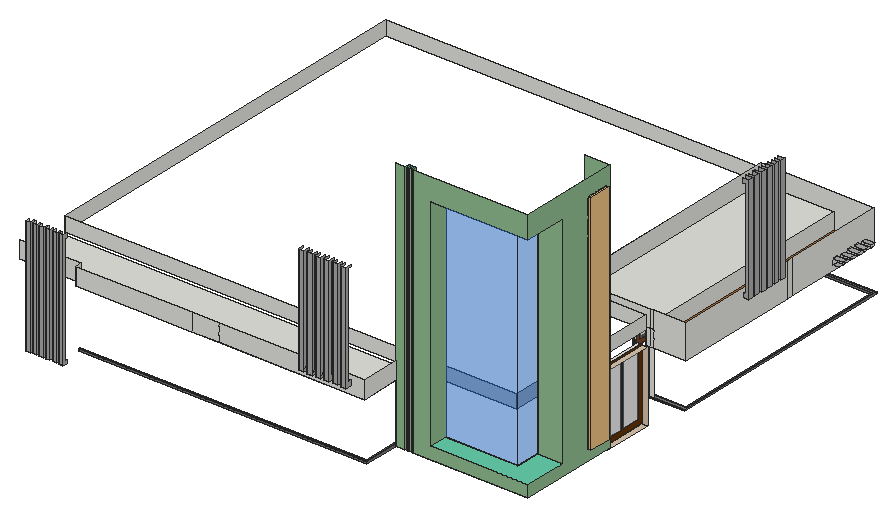
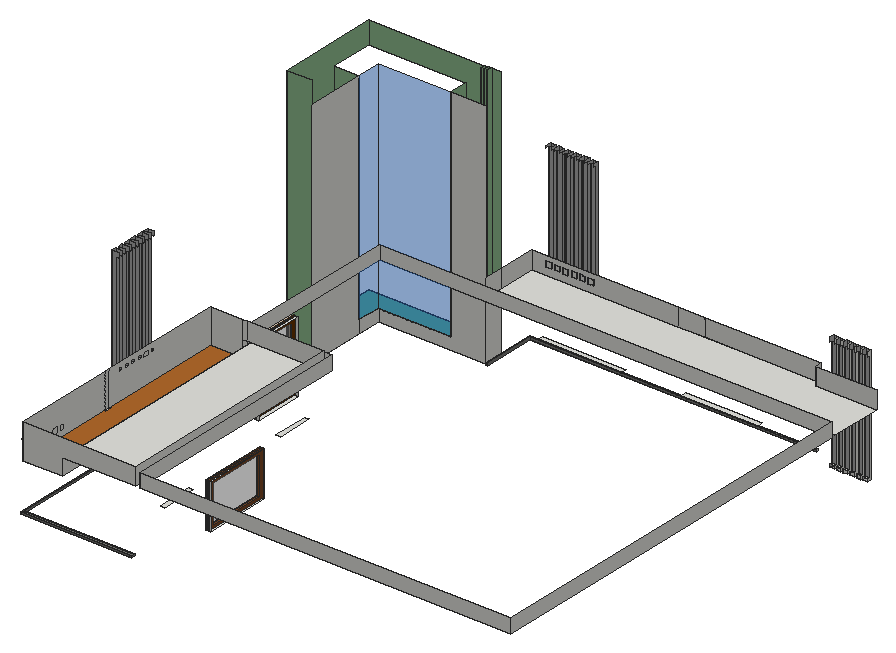
# SketchUp Ruby script. Lengths in inches.
U = 1.inch
M = Sketchup.active_model
def pt(a) = Geom::Point3d.new(a.map { |v| v * U })
def face(e, loops, mat)
  f = e.add_face(loops[0].map { |a| pt(a) })
  loops[1..].each { |l| e.add_face(l.map { |a| pt(a) }).erase! }
  f.material = f.back_material = mat if mat
  f
end
# faces: each face lists its corners as indices into pts; further lists are holes
def faces(e, pts, list, mat = nil) = list.each { |f| face(e, (f[0].is_a?(Array) ? f : [f]).map { |l| l.map { |i| pts[i] } }, mat) }
# xy, xz, yz: faces in a plane at the given z, y or x. An outline is a flat list of corners, or four numbers for a rectangle; further outlines are holes
def ring(l) = l.size == 4 ? [[l[0], l[1]], [l[2], l[1]], [l[2], l[3]], [l[0], l[3]]] : l.each_slice(2).to_a
def flat(e, list, mat, &to3) = list.each { |f| face(e, (f[0].is_a?(Array) ? f : [f]).map { |l| ring(l).map { |u, v| to3.(u, v) } }, mat) }
def xy(e, z, list, mat = nil) = flat(e, list, mat) { |x, y| [x, y, z] }
def xz(e, y, list, mat = nil) = flat(e, list, mat) { |x, z| [x, y, z] }
def yz(e, x, list, mat = nil) = flat(e, list, mat) { |y, z| [x, y, z] }
def lines(e, pts, list) = list.each { |a, b| e.add_line(pt(pts[a]), pt(pts[b])) }
# prism: a flat outline (further loops are holes) pulled along v
def prism(e, loops, v, mat = nil)
  f = face(e, loops, mat); d = Geom::Vector3d.new(v.map { |x| x * U })
  f.pushpull(f.normal.samedirection?(d) ? d.length : -d.length)
end
def box(e, o, s, mat = nil) = prism(e, [[o, [o[0] + s[0], o[1], o[2]], [o[0] + s[0], o[1] + s[1], o[2]], [o[0], o[1] + s[1], o[2]]]], [0, 0, s[2]], mat)
def at(x, y, z, deg = 0) = Geom::Transformation.translation(pt([x, y, z])) * Geom::Transformation.rotation(ORIGIN, Z_AXIS, deg.degrees)
def axes(o, x, y, z) = Geom::Transformation.new([*x, 0, *y, 0, *z, 0, *pt(o).to_a, 1])
def part(name) = M.definitions.add(name)
# library, detail: a bought-in or finely detailed component or shape, given as its bounding box
def library(name, o, s) = part(name).tap { |d| box(d.entities, o, s) }
def detail(e, o, s) = box(e.add_group.entities, o, s)
def put(e, d, t, mat = nil) = e.add_instance(d, t).tap { |i| i.material = mat if mat }
def group(e, t, mat = nil) = e.add_group.tap { |g| g.transformation = t; g.material = mat if mat }.entities
root = M.entities
M.materials.add("[0072_DarkSeaGreen]").color = [143, 188, 143]
M.materials.add("[0086_MediumAquamarine]").color = [102, 205, 170]
M.materials.add("[Blinds Cellular White]").color = [216, 195, 171]
M.materials.add("[Color C08]").color = [102, 51, 0]
M.materials.add("[Color E02]").color = [255, 255, 153]
M.materials.add("[Color M03]").color = [170, 170, 170]
M.materials.add("[Metal Seamed]").color = [118, 119, 115]
M.materials.add("[Translucent Glass Gray]").color = [128, 128, 128]
M.materials["[Translucent Glass Gray]"].alpha = 0.5
M.materials.add("[Translucent Glass Sky Reflection]").color = [37, 119, 229]
M.materials["[Translucent Glass Sky Reflection]"].alpha = 0.52
M.materials.add("[Wood Bamboo]").color = [177, 105, 43]
M.materials.add("[Wood Veneer 01]").color = [120, 70, 37]
c1 = part("Group\#4")
xy(c1.entities,0,[[0,0,92.3125,1154.125]],"[Wood Veneer 01]")
xy(c1.entities,74.3,[[0,74.3,92.3125,1079.83]],"[Wood Veneer 01]")
xy(c1.entities,936.58,[[0,74.3,92.3125,1079.83]],"[Wood Veneer 01]")
xy(c1.entities,1010.875,[[0,0,92.3125,1154.125]],"[Wood Veneer 01]")
xz(c1.entities,0,[[0,0,92.3125,1010.875]],"[Wood Veneer 01]")
xz(c1.entities,74.3,[[0,74.3,92.3125,936.58]],"[Wood Veneer 01]")
xz(c1.entities,1079.83,[[0,74.3,92.3125,936.58]],"[Wood Veneer 01]")
xz(c1.entities,1154.125,[[0,0,92.3125,1010.875]],"[Wood Veneer 01]")
yz(c1.entities,0,[[[0,0,1154.125,1010.875],[74.3,74.3,1079.83,936.58]]],"[Wood Veneer 01]")
yz(c1.entities,92.3125,[[74.3,74.3,1079.83,936.58]],"[Translucent Glass Gray]")
yz(c1.entities,92.3125,[[[0,0,1154.125,1010.875],[74.3,74.3,1079.83,936.58]]],"[Wood Veneer 01]")
c2 = part("Group\#1")
xy(c2.entities,0,[[0,0,56.25,1.4375]],"[Color C08]")
xy(c2.entities,4.61,[[4.61,0,27.19,1.4375],[28.74,0,51.64,1.4375]],"[Color C08]")
xy(c2.entities,68.58,[[4.61,0,27.19,1.4375],[28.74,0,51.64,1.4375]],"[Color C08]")
xy(c2.entities,73.1875,[[0,0,56.25,1.4375]],"[Color C08]")
xz(c2.entities,0,[[[0,0,56.25,73.1875],[28.74,4.61,51.64,68.58],[4.61,4.61,27.19,68.58]]],"[Color C08]")
xz(c2.entities,0,[[4.61,4.61,27.19,68.58],[28.74,4.61,51.64,68.58]],"[Translucent Glass Gray]")
xz(c2.entities,1.4375,[[[0,0,56.25,73.1875],[28.74,4.61,51.64,68.58],[4.61,4.61,27.19,68.58]]],"[Color C08]")
yz(c2.entities,0,[[0,0,1.4375,73.1875]],"[Color C08]")
yz(c2.entities,4.61,[[0,4.61,1.4375,68.58]],"[Color C08]")
yz(c2.entities,27.19,[[0,4.61,1.4375,68.58]],"[Color C08]")
yz(c2.entities,28.74,[[0,4.61,1.4375,68.58]],"[Color C08]")
yz(c2.entities,51.64,[[0,4.61,1.4375,68.58]],"[Color C08]")
yz(c2.entities,56.25,[[0,0,1.4375,73.1875]],"[Color C08]")
c3 = library("D E S H M U K H",[0.1875,0,0],[29.86,305.5625,4])
xy(root,172.67,[[554.1875,452.44,560.1875,543.38]])
xy(root,173.05,[[663.6875,257.99,669.6875,324.49]])
xy(root,173.05,[[669.6875,257.99,676.75,324.49]],"[Blinds Cellular White]")
xy(root,180.1,[[70.8125,30.88,76.8125,36.13],[79.75,30.88,85.75,36.07],[88.6875,30.88,94.6875,35.88],[97.625,30.88,103.625,36.25],[106.5625,30.88,112.5625,36.13],
  [115.375,30.88,121.375,36.13]],"[Color M03]")
xy(root,184.32,[[70.8125,33.13,76.8125,36.13],[79.75,33.13,85.75,36.07],[88.6875,33.13,94.6875,35.88],[97.625,33.13,103.625,36.25],[106.5625,33.13,112.5625,36.13],
  [115.375,33.13,121.375,36.13]])
xy(root,194,[[663.6875,344.5,663.6875,349.5,708.8125,349.5,708.8125,663.625,560.1875,663.625,560.1875,668.5625,711.3125,668.5625,711.3125,344.5]],"[Metal Seamed]")
xy(root,196,[[663.6875,344.5,711.3125,344.5,711.3125,668.5625,560.1875,668.5625,560.1875,663.625,708.8125,663.625,708.8125,349.5,663.6875,349.5]],"[Metal Seamed]")
xy(root,197.41,[[133.9375,41,133.9375,43,521.9375,43,521.9375,114.75,523.9375,114.75,523.9375,41]])
xy(root,198.5,[[524.8125,89.3125,524.8125,114.75,669.6875,114.75,669.6875,228.1875,703.5625,228.1875,703.5625,89.3125,547.08,89.3125,547.08,94.9375,545.625,94.9375,545.625,89.3125,542.52,89.3125,542.52,94.9375,541.0625,94.9375,541.0625,89.3125,538.83,89.3125,538.83,94.9375,537.375,94.9375,537.375,89.3125]],"[0072_DarkSeaGreen]")
xy(root,200.41,[[133.9375,41,523.9375,41,523.9375,114.75,521.9375,114.75,521.9375,43,133.9375,43]],"[Metal Seamed]")
xy(root,214.64,[[571.375,89.3125,703.5625,89.3125,703.5625,147.3125,669.6875,147.3125,669.6875,114.75,571.375,114.75]],"[0086_MediumAquamarine]")
xy(root,233.42,[[554.1875,452.44,560.1875,543.38]])
xy(root,236,[[554.1875,376.72,560.1875,424.72]])
xy(root,236.0625,[[554.1875,572.375,560.1875,620.375]])
xy(root,255.6875,[[710.9375,516.39,713,523.93]])
xy(root,255.6875,[[659.09,344.5,659.09,662.5625,713,662.5625,713,523.93,710.9375,523.93,710.9375,516.39,713,516.39,713,344.5]],"[Wood Bamboo]")
xy(root,257.77,[[150.78,114.75,253.85,120.75]])
xy(root,257.8125,[[335.54,114.75,448.04,120.75]])
xy(root,263.23,[[713,592.7,721.8125,600.33],[713,604.52,721.8125,612.14],[713,616.33,721.8125,623.95],[713,628.14,721.8125,635.77],[713,639.95,721.8125,647.58]],"[Color M03]")
xy(root,268.99,[[663.6875,257.99,669.6875,324.49]])
xy(root,268.99,[[669.6875,257.99,676.75,324.49]],"[Blinds Cellular White]")
xy(root,270.86,[[713,592.7,726.25,600.33],[713,604.52,726.25,612.14],[713,616.33,726.25,623.95],[713,628.14,726.25,635.77],[713,639.95,726.25,647.58]],"[Color M03]")
xy(root,278,[[133.9375,36.13,133.9375,45.16,51.8125,45.16,51.8125,114.75,524.8125,114.75,524.8125,36.13],[560.1875,344.5,659.09,662.5625]])
xy(root,287.98,[[441.9,28.63,448.9,36.13],[453.28,28.63,460.28,36.13],[464.65,28.63,471.65,36.13],[476.03,28.63,483.03,36.13],[487.4,28.63,494.4,36.13],
  [498.78,28.63,505.78,36.13]],"[Color M03]")
xy(root,291.22,[[713,439.9375,721.8125,446.375],[712.75,450.75,721.8125,457.1875],[713,461.5625,721.8125,468],[713,472.375,721.8125,478.8125],[713,483.1875,721.8125,489.625],
  [713,494,721.8125,500.4375]],"[Color M03]")
xy(root,294.98,[[441.9,31.63,448.9,36.13],[453.28,31.63,460.28,36.13],[464.65,31.63,471.65,36.13],[476.03,31.63,483.03,36.13],[487.4,31.63,494.4,36.13],
  [498.78,31.63,505.78,36.13]])
xz(root,28.63,[[441.9,287.98,448.9,434.85],[453.28,287.98,460.28,434.85],[464.65,287.98,471.65,434.85],[476.03,287.98,483.03,434.85],[487.4,287.98,494.4,434.85],
  [498.78,287.98,505.78,434.85]],"[Color M03]")
xz(root,30.88,[[70.8125,180.1,76.8125,338.1],[79.75,180.1,85.75,338.1],[88.6875,180.1,94.6875,338.1],[97.625,180.1,103.625,338.1],[106.5625,180.1,112.5625,338.1],
  [115.375,180.1,121.375,338.1]],"[Color M03]")
xz(root,31.63,[[441.9,294.98,448.9,432.27],[453.28,294.98,460.28,432.27],[464.65,294.98,471.65,432.27],[476.03,294.98,483.03,432.27],[487.4,294.98,494.4,432.27],
  [498.78,294.98,505.78,432.27]],"[Color M03]")
xz(root,33.13,[[70.8125,184.32,76.8125,332.1],[79.75,184.32,85.75,332.1],[88.6875,184.32,94.6875,332.1],[97.625,184.32,103.625,332.1],[106.5625,184.32,112.5625,332.1],
  [115.375,184.32,121.375,332.1]],"[Color M03]")
xz(root,35.88,[[88.6875,180.1,94.6875,184.32]])
xz(root,36.07,[[79.75,180.1,85.75,184.32]])
xz(root,36.13,[[133.9375,278,291.33,302],[291.33,278,327.08,302],[[327.08,278,524.8125,302],[498.78,287.98,505.78,294.98],[487.4,287.98,494.4,294.98],[476.03,287.98,483.03,294.98],[464.65,287.98,471.65,294.98],[453.28,287.98,460.28,294.98],[441.9,287.98,448.9,294.98]],[441.9,287.98,448.9,294.98],[453.28,287.98,460.28,294.98],
  [464.65,287.98,471.65,294.98],[476.03,287.98,483.03,294.98],[487.4,287.98,494.4,294.98],[498.78,287.98,505.78,294.98]])
xz(root,36.25,[[97.625,180.1,103.625,184.32]])
xz(root,41,[[133.9375,197.41,523.9375,200.41]],"[Metal Seamed]")
xz(root,43,[[133.9375,197.41,521.9375,200.41]],"[Metal Seamed]")
xz(root,45.16,[[51.8125,278,133.9375,302]])
xz(root,89.3125,[[524.8125,198.5,537.375,541.0625],[538.83,198.5,541.0625,541.0625],[542.52,198.5,545.625,541.0625],[547.08,198.5,703.5625,198.5,703.5625,214.64,571.375,214.64,571.375,511.125,703.5625,511.125,703.5625,541.0625,547.08,541.0625]],"[0072_DarkSeaGreen]")
xz(root,94.9375,[[537.375,198.5,538.83,541.0625],[541.0625,198.5,542.52,541.0625],[545.625,198.5,547.08,541.0625]],"[0072_DarkSeaGreen]")
xz(root,114.75,[[521.9375,197.41,523.9375,200.41],[524.8125,198.5,524.8125,511.125,571.375,511.125,571.375,214.64,669.6875,214.64,669.6875,198.5]])
xz(root,114.75,[[571.375,214.64,669.6875,511.125]],"[Translucent Glass Sky Reflection]")
xz(root,120.75,[[51.8125,278,663.6875,297]])
xz(root,147.3125,[[669.6875,214.64,703.5625,511.125]],"[0072_DarkSeaGreen]")
xz(root,228.1875,[[669.6875,198.5,703.5625,541.0625]],"[0072_DarkSeaGreen]")
xz(root,257.99,[[663.6875,173.05,669.6875,268.99]])
xz(root,257.99,[[669.6875,173.05,676.75,268.99]],"[Blinds Cellular White]")
xz(root,324.49,[[663.6875,173.05,669.6875,268.99]])
xz(root,324.49,[[669.6875,173.05,676.75,268.99]],"[Blinds Cellular White]")
xz(root,338.5,[[554.1875,278,663.6875,297]])
xz(root,344.5,[[663.6875,196,669.6875,255.6875],[659.09,255.6875,663.6875,278],[663.6875,255.6875,669.6875,278],[669.6875,255.6875,713,302],[560.1875,278,663.6875,302],
  [663.6875,278,669.6875,302]])
xz(root,344.5,[[663.6875,194,669.6875,196],[669.6875,194,711.3125,196]],"[Metal Seamed]")
xz(root,349.5,[[663.6875,194,708.8125,196]],"[Metal Seamed]")
xz(root,439.9375,[[713,291.22,721.8125,291.22,721.8125,436.0625,713,436.0625,713,429.625,717.1875,429.625,717.1875,296.2,713,296.2]],"[Color M03]")
xz(root,446.375,[[713,291.22,713,296.2,717.1875,296.2,717.1875,429.625,713,429.625,713,436.0625,721.8125,436.0625,721.8125,291.22]],"[Color M03]")
xz(root,450.75,[[712.75,291.22,721.8125,291.22,721.8125,436.0625,713,436.0625,713,429.625,717.1875,429.625,717.1875,296.2,712.75,296.2]],"[Color M03]")
xz(root,452.44,[[554.1875,172.67,560.1875,233.42]])
xz(root,457.1875,[[712.75,291.22,712.75,296.2,717.1875,296.2,717.1875,429.625,713,429.625,713,436.0625,721.8125,436.0625,721.8125,291.22]],"[Color M03]")
xz(root,461.5625,[[713,291.22,721.8125,291.22,721.8125,436.0625,713,436.0625,713,429.625,717.1875,429.625,717.1875,296.2,713,296.2]],"[Color M03]")
xz(root,468,[[713,291.22,713,296.2,717.1875,296.2,717.1875,429.625,713,429.625,713,436.0625,721.8125,436.0625,721.8125,291.22]],"[Color M03]")
xz(root,472.375,[[713,291.22,721.8125,291.22,721.8125,436.0625,713,436.0625,713,429.625,717.1875,429.625,717.1875,296.2,713,296.2]],"[Color M03]")
xz(root,478.8125,[[713,291.22,713,296.2,717.1875,296.2,717.1875,429.625,713,429.625,713,436.0625,721.8125,436.0625,721.8125,291.22]],"[Color M03]")
xz(root,483.1875,[[713,291.22,721.8125,291.22,721.8125,436.0625,713,436.0625,713,429.625,717.1875,429.625,717.1875,296.2,713,296.2]],"[Color M03]")
xz(root,489.625,[[713,291.22,713,296.2,717.1875,296.2,717.1875,429.625,713,429.625,713,436.0625,721.8125,436.0625,721.8125,291.22]],"[Color M03]")
xz(root,494,[[713,291.22,721.8125,291.22,721.8125,436.0625,713,436.0625,713,429.625,717.1875,429.625,717.1875,296.2,713,296.2]],"[Color M03]")
xz(root,500.4375,[[713,291.22,713,296.2,717.1875,296.2,717.1875,429.625,713,429.625,713,436.0625,721.8125,436.0625,721.8125,291.22]],"[Color M03]")
xz(root,543.38,[[554.1875,172.67,560.1875,233.42]])
xz(root,662.5625,[[659.09,255.6875,659.09,278,560.1875,278,560.1875,302,713,302,713,255.6875],[51.8125,278,554.1875,297]])
xz(root,663.625,[[560.1875,194,708.8125,196]],"[Metal Seamed]")
xz(root,668.5625,[[560.1875,194,711.3125,196]],"[Metal Seamed]")
yz(root,51.8125,[[120.75,278,662.5625,297]])
yz(root,70.8125,[[30.88,180.1,30.88,338.1,36.13,338.1,36.13,332.1,33.13,332.1,33.13,184.32,36.13,184.32,36.13,180.1]])
yz(root,76.8125,[[30.88,180.1,36.13,180.1,36.13,184.32,33.13,184.32,33.13,332.1,36.13,332.1,36.13,338.1,30.88,338.1]],"[Color M03]")
yz(root,79.75,[[30.88,180.1,30.88,338.1,36.13,338.1,36.13,332.1,33.13,332.1,33.13,184.32,36.07,184.32,36.07,180.1]])
yz(root,85.75,[[30.88,180.1,36.07,180.1,36.07,184.32,33.13,184.32,33.13,332.1,36.13,332.1,36.13,338.1,30.88,338.1]],"[Color M03]")
yz(root,88.6875,[[30.88,180.1,30.88,338.1,36.13,338.1,36.13,332.1,33.13,332.1,33.13,184.32,35.88,184.32,35.88,180.1]])
yz(root,94.6875,[[30.88,180.1,35.88,180.1,35.88,184.32,33.13,184.32,33.13,332.1,36.13,332.1,36.13,338.1,30.88,338.1]],"[Color M03]")
yz(root,97.625,[[30.88,180.1,30.88,338.1,36.13,338.1,36.13,332.1,33.13,332.1,33.13,184.32,36.25,184.32,36.25,180.1]])
yz(root,103.625,[[30.88,180.1,36.25,180.1,36.25,184.32,33.13,184.32,33.13,332.1,36.13,332.1,36.13,338.1,30.88,338.1]],"[Color M03]")
yz(root,106.5625,[[30.88,180.1,30.88,338.1,36.13,338.1,36.13,332.1,33.13,332.1,33.13,184.32,36.13,184.32,36.13,180.1]])
yz(root,112.5625,[[30.88,180.1,36.13,180.1,36.13,184.32,33.13,184.32,33.13,332.1,36.13,332.1,36.13,338.1,30.88,338.1]],"[Color M03]")
yz(root,115.375,[[30.88,180.1,30.88,338.1,36.13,338.1,36.13,332.1,33.13,332.1,33.13,184.32,36.13,184.32,36.13,180.1]])
yz(root,121.375,[[30.88,180.1,36.13,180.1,36.13,184.32,33.13,184.32,33.13,332.1,36.13,332.1,36.13,338.1,30.88,338.1]],"[Color M03]")
yz(root,133.9375,[[41,197.41,43,200.41],[36.13,278,45.16,302]])
yz(root,441.9,[[28.63,287.98,28.63,434.85,36.13,434.85,36.13,432.27,31.63,432.27,31.63,294.98,36.13,294.98,36.13,287.98]],"[Color M03]")
yz(root,448.9,[[28.63,287.98,36.13,287.98,36.13,294.98,31.63,294.98,31.63,291.48,28.63,291.48],[28.63,291.48,31.63,291.48,31.63,432.27,36.13,432.27,36.13,434.85,28.63,434.85]],"[Color M03]")
yz(root,453.28,[[28.63,287.98,28.63,434.85,36.07,434.85,36.07,432.27,31.63,432.27,31.63,294.98,36.13,294.98,36.13,287.98]],"[Color M03]")
yz(root,460.28,[[28.63,287.98,36.13,287.98,36.13,294.98,31.63,294.98,31.63,291.48,28.63,291.48],[28.63,291.48,31.63,291.48,31.63,432.27,36.07,432.27,36.07,434.85,28.63,434.85]],"[Color M03]")
yz(root,464.65,[[28.63,287.98,28.63,434.85,36.13,434.85,36.13,432.27,31.63,432.27,31.63,294.98,36.13,294.98,36.13,287.98]],"[Color M03]")
yz(root,471.65,[[28.63,287.98,36.13,287.98,36.13,294.98,31.63,294.98,31.63,291.48,28.63,291.48],[28.63,291.48,31.63,291.48,31.63,432.27,36.13,432.27,36.13,434.85,28.63,434.85]],"[Color M03]")
yz(root,476.03,[[28.63,287.98,28.63,434.85,36,434.85,36,432.27,31.63,432.27,31.63,294.98,36.13,294.98,36.13,287.98]],"[Color M03]")
yz(root,483.03,[[28.63,287.98,36.13,287.98,36.13,294.98,31.63,294.98,31.63,432.27,36,432.27,36,434.85,28.63,434.85]],"[Color M03]")
yz(root,487.4,[[28.63,287.98,28.63,434.85,36.13,434.85,36.13,432.27,31.63,432.27,31.63,294.98,36.13,294.98,36.13,287.98]],"[Color M03]")
yz(root,494.4,[[28.63,287.98,36.13,287.98,36.13,294.98,31.63,294.98,31.63,432.27,36.13,432.27,36.13,434.85,28.63,434.85]],"[Color M03]")
yz(root,498.78,[[28.63,287.98,28.63,434.85,36.13,434.85,36.13,432.27,31.63,432.27,31.63,294.98,36.13,294.98,36.13,287.98]],"[Color M03]")
yz(root,505.78,[[28.63,287.98,36.13,287.98,36.13,294.98,31.63,294.98,31.63,432.27,36.13,432.27,36.13,434.85,28.63,434.85]],"[Color M03]")
yz(root,521.9375,[[43,197.41,114.75,200.41]],"[Metal Seamed]")
yz(root,523.9375,[[41,197.41,114.75,200.41]],"[Metal Seamed]")
yz(root,524.8125,[[89.3125,198.5,114.75,278],[36.13,278,89.3125,302],[89.3125,278,114.75,302]])
yz(root,537.375,[[89.3125,198.5,94.9375,541.0625]],"[0072_DarkSeaGreen]")
yz(root,538.83,[[89.3125,198.5,94.9375,541.0625]],"[0086_MediumAquamarine]")
yz(root,541.0625,[[89.3125,198.5,94.9375,541.0625]],"[0072_DarkSeaGreen]")
yz(root,542.52,[[89.3125,198.5,94.9375,541.0625]],"[0086_MediumAquamarine]")
yz(root,545.625,[[89.3125,198.5,94.9375,541.0625]],"[0072_DarkSeaGreen]")
yz(root,547.08,[[89.3125,198.5,94.9375,541.0625]],"[0072_DarkSeaGreen]")
yz(root,554.1875,[[338.5,278,662.5625,297]])
yz(root,560.1875,[[344.5,278,662.5625,302]])
yz(root,560.1875,[[663.625,194,668.5625,196]],"[Metal Seamed]")
yz(root,571.375,[[89.3125,214.64,114.75,511.125]],"[0072_DarkSeaGreen]")
yz(root,659.09,[[344.5,255.6875,662.5625,278]])
yz(root,663.6875,[[120.75,278,338.5,297]])
yz(root,663.6875,[[344.5,194,349.5,196]],"[Metal Seamed]")
yz(root,669.6875,[[114.75,198.5,147.3125,214.64],[147.3125,198.5,228.1875,511.125]])
yz(root,669.6875,[[114.75,214.64,147.3125,511.125]],"[Translucent Glass Sky Reflection]")
yz(root,703.5625,[[89.3125,198.5,228.1875,198.5,228.1875,541.0625,89.3125,541.0625,89.3125,511.125,147.3125,511.125,147.3125,214.64,89.3125,214.64]],"[0072_DarkSeaGreen]")
yz(root,708.8125,[[349.5,194,663.625,196]],"[Metal Seamed]")
yz(root,711.3125,[[344.5,194,668.5625,196]],"[Metal Seamed]")
yz(root,712.75,[[450.75,291.22,457.1875,296.2]])
yz(root,713,[[[344.5,255.6875,516.39,302],[494,291.22,500.4375,296.2],[483.1875,291.22,489.625,296.2],[472.375,291.22,478.8125,296.2],[461.5625,291.22,468,296.2],[439.9375,291.22,446.375,296.2]],[516.39,255.6875,523.93,302],[[523.93,255.6875,662.5625,302],[639.95,263.23,647.58,270.86],[628.14,263.23,635.77,270.86],[616.33,263.23,623.95,270.86],[604.52,263.23,612.14,270.86],[592.7,263.23,600.33,270.86]],[592.7,263.23,600.33,270.86],[604.52,263.23,612.14,270.86],
  [616.33,263.23,623.95,270.86],[628.14,263.23,635.77,270.86],[639.95,263.23,647.58,270.86]])
yz(root,721.8125,[[439.9375,291.22,446.375,436.0625],[450.75,291.22,457.1875,436.0625],[461.5625,291.22,468,436.0625],[472.375,291.22,478.8125,436.0625],[483.1875,291.22,489.625,436.0625],
  [494,291.22,500.4375,436.0625]],"[Color M03]")
p = [[453.28,31.63,291.48],[460.28,31.63,291.48]]
lines(root,p,[[0,1]])
put(root,c1,axes([556.02,452.44,172.67],[0.03924,0,0],[0,0.07879,0],[0,0,0.0601]))
put(root,c2,axes([669.6875,257.99,173.55],[0,1.18222,0],[-1,0,0],[0,0,1.31085]))
put(root,c3,axes([703.5625,190.06,213.14],[0,1,0],[0,0,1],[1,0,0]),"[Color E02]")
